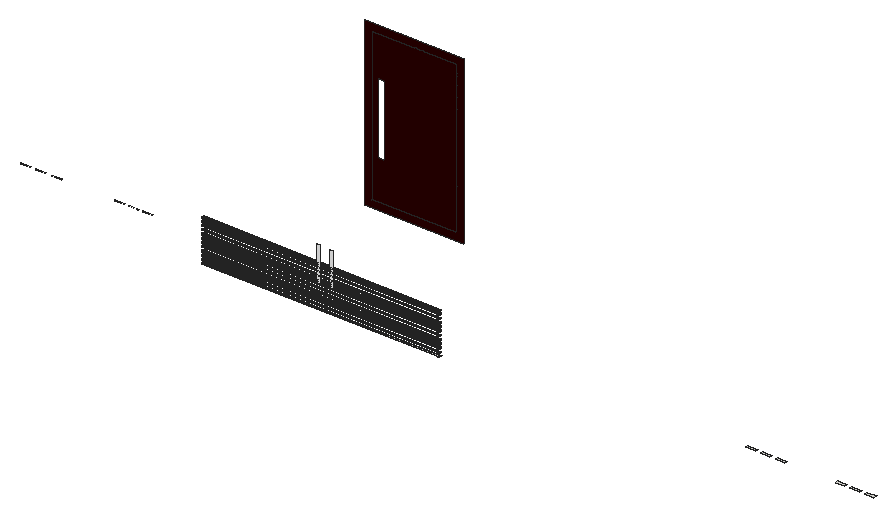
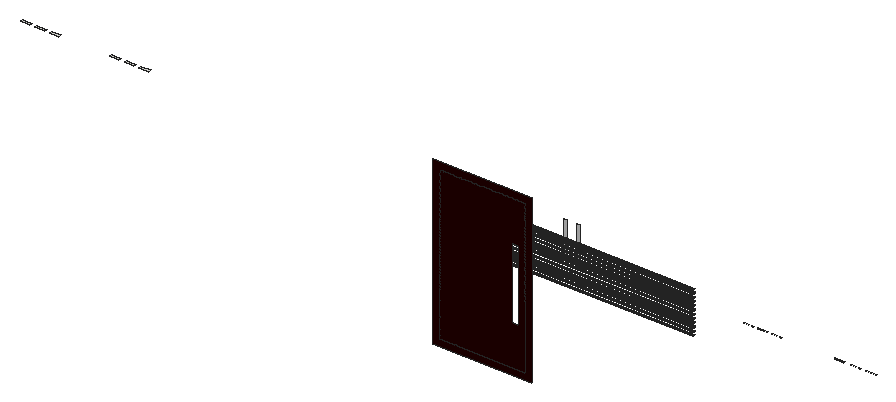
# SketchUp Ruby script. Lengths in inches.
U = 1.inch
M = Sketchup.active_model
def pt(a) = Geom::Point3d.new(a.map { |v| v * U })
def face(e, loops, mat)
  f = e.add_face(loops[0].map { |a| pt(a) })
  loops[1..].each { |l| e.add_face(l.map { |a| pt(a) }).erase! }
  f.material = f.back_material = mat if mat
  f
end
# faces: each face lists its corners as indices into pts; further lists are holes
def faces(e, pts, list, mat = nil) = list.each { |f| face(e, (f[0].is_a?(Array) ? f : [f]).map { |l| l.map { |i| pts[i] } }, mat) }
# xy, xz, yz: faces in a plane at the given z, y or x. An outline is a flat list of corners, or four numbers for a rectangle; further outlines are holes
def ring(l) = l.size == 4 ? [[l[0], l[1]], [l[2], l[1]], [l[2], l[3]], [l[0], l[3]]] : l.each_slice(2).to_a
def flat(e, list, mat, &to3) = list.each { |f| face(e, (f[0].is_a?(Array) ? f : [f]).map { |l| ring(l).map { |u, v| to3.(u, v) } }, mat) }
def xy(e, z, list, mat = nil) = flat(e, list, mat) { |x, y| [x, y, z] }
def xz(e, y, list, mat = nil) = flat(e, list, mat) { |x, z| [x, y, z] }
def yz(e, x, list, mat = nil) = flat(e, list, mat) { |y, z| [x, y, z] }
def lines(e, pts, list) = list.each { |a, b| e.add_line(pt(pts[a]), pt(pts[b])) }
# prism: a flat outline (further loops are holes) pulled along v
def prism(e, loops, v, mat = nil)
  f = face(e, loops, mat); d = Geom::Vector3d.new(v.map { |x| x * U })
  f.pushpull(f.normal.samedirection?(d) ? d.length : -d.length)
end
def box(e, o, s, mat = nil) = prism(e, [[o, [o[0] + s[0], o[1], o[2]], [o[0] + s[0], o[1] + s[1], o[2]], [o[0], o[1] + s[1], o[2]]]], [0, 0, s[2]], mat)
def at(x, y, z, deg = 0) = Geom::Transformation.translation(pt([x, y, z])) * Geom::Transformation.rotation(ORIGIN, Z_AXIS, deg.degrees)
def axes(o, x, y, z) = Geom::Transformation.new([*x, 0, *y, 0, *z, 0, *pt(o).to_a, 1])
def part(name) = M.definitions.add(name)
# library, detail: a bought-in or finely detailed component or shape, given as its bounding box
def library(name, o, s) = part(name).tap { |d| box(d.entities, o, s) }
def detail(e, o, s) = box(e.add_group.entities, o, s)
def put(e, d, t, mat = nil) = e.add_instance(d, t).tap { |i| i.material = mat if mat }
def group(e, t, mat = nil) = e.add_group.tap { |g| g.transformation = t; g.material = mat if mat }.entities
root = M.entities
M.materials.add("[0022_Maroon]").color = [43, 0, 0]
M.materials.add("[0128_White]").color = [255, 255, 255]
xy(root,190.5,[[15.39,67,40.95,69],[55.2,67,80.76,69],[98.33,67,123.89,69],[262.89,67,288.45,69],[300.83,67,326.39,69],
  [336.83,67,362.39,69]])
xy(root,214.5,[[1949.82,36,1975.38,43],[1988.38,36,2013.94,43],[2028.13,36,2053.69,43],[2185.76,36,2211.32,43],[2224.38,36,2249.94,43],
  [2262.44,36,2288.01,43]])
xz(root,71.03,[[791.39,180.6,799.64,271.47],[827.39,180.6,835.64,271.47]],"[0128_White]")
xz(root,455.71,[[[611.72,132,872.28,567.56],[629.72,150,854.28,549.56]],[[629.72,150,854.28,549.56],[645.54,254.24,665.16,443.24]]],"[0022_Maroon]")
p = [[489.6,72.78,119.6875],[489.6,72.58,119.2],[1116.35,72.58,119.2],[1116.35,72.78,119.6875],[489.6,76.45,119.2],[489.6,76.25,119.6875],
  [1116.35,76.25,119.6875],[1116.35,76.45,119.2],[489.6,73.1,120.1],[1116.35,73.1,120.1],[489.6,75.93,120.1],[1116.35,75.93,120.1],
  [489.6,73.52,120.42],[1116.35,73.52,120.42],[489.6,75.52,120.42],[1116.35,75.52,120.42],[489.6,74,120.62],[1116.35,74,120.62],
  [489.6,75.03,120.62],[1116.35,75.03,120.62],[489.6,74.52,120.6875],[1116.35,74.52,120.6875],[489.6,74,126.75],[489.6,74.52,126.6875],
  [1116.05,74.52,126.6875],[1116.05,74,126.75],[489.6,75.03,126.75],[1116.05,75.03,126.75],[489.6,73.52,126.95],[1116.05,73.52,126.95],
  [489.6,75.52,126.95],[1116.05,75.52,126.95],[489.6,73.1,127.27],[1116.05,73.1,127.27],[489.6,75.93,127.27],[1116.05,75.93,127.27],
  [489.6,72.78,127.6875],[1116.05,72.78,127.6875],[489.6,76.25,127.6875],[1116.05,76.25,127.6875],[489.6,72.58,128.17],[1116.05,72.58,128.17],
  [489.6,76.45,128.17],[1116.05,76.45,128.17],[489.6,72.52,128.6875],[1116.05,72.52,128.6875],[489.6,76.52,128.6875],[1116.05,76.52,128.6875],
  [489.6,72.58,129.2],[1116.05,72.58,129.2],[489.6,76.45,129.2],[1116.05,76.45,129.2],[489.6,72.78,129.6875],[1116.05,72.78,129.6875],
  [489.6,76.25,129.6875],[1116.05,76.25,129.6875],[489.6,73.1,130.1],[1116.05,73.1,130.1],[489.6,75.93,130.1],[1116.05,75.93,130.1],
  [489.6,73.52,130.42],[1116.05,73.52,130.42],[489.6,75.52,130.42],[1116.05,75.52,130.42],[489.6,74,130.62],[1116.05,74,130.62],
  [489.6,75.03,130.62],[1116.05,75.03,130.62],[489.6,74.52,130.6875],[1116.05,74.52,130.6875],[489.6,74,136.75],[489.6,74.52,136.6875],
  [1116.05,74.52,136.6875],[1116.05,74,136.75],[489.6,75.03,136.75],[1116.05,75.03,136.75],[489.6,73.52,136.95],[1116.05,73.52,136.95],
  [489.6,75.52,136.95],[1116.05,75.52,136.95],[489.6,73.1,137.27],[1116.05,73.1,137.27],[489.6,75.93,137.27],[1116.05,75.93,137.27],
  [489.6,72.78,137.6875],[1116.05,72.78,137.6875],[489.6,76.25,137.6875],[1116.05,76.25,137.6875],[489.6,72.58,138.17],[1116.05,72.58,138.17],
  [489.6,76.45,138.17],[1116.05,76.45,138.17],[489.6,72.52,138.6875],[1116.05,72.52,138.6875],[489.6,76.52,138.6875],[1116.05,76.52,138.6875],
  [489.6,72.58,139.2],[1116.05,72.58,139.2],[489.6,76.45,139.2],[1116.05,76.45,139.2],[489.6,72.78,139.6875],[1116.05,72.78,139.6875],
  [489.6,76.25,139.6875],[1116.05,76.25,139.6875],[489.6,73.1,140.1],[1116.05,73.1,140.1],[489.6,75.93,140.1],[1116.05,75.93,140.1],
  [489.6,73.52,140.42],[1116.05,73.52,140.42],[489.6,75.52,140.42],[1116.05,75.52,140.42],[489.6,74,140.62],[1116.05,74,140.62],
  [489.6,75.03,140.62],[1116.05,75.03,140.62],[489.6,74.52,140.6875],[1116.05,74.52,140.6875],[489.6,74,146.75],[489.6,74.52,146.6875],
  [1116.05,74.52,146.6875],[1116.05,74,146.75],[489.6,75.03,146.75],[1116.05,75.03,146.75],[489.6,73.52,146.95],[1116.05,73.52,146.95],
  [489.6,75.52,146.95],[1116.05,75.52,146.95],[489.6,73.1,147.27],[1116.05,73.1,147.27],[489.6,75.93,147.27],[1116.05,75.93,147.27],
  [489.6,72.78,147.6875],[1116.05,72.78,147.6875],[489.6,76.25,147.6875],[1116.05,76.25,147.6875],[489.6,72.58,148.17],[1116.05,72.58,148.17],
  [489.6,76.45,148.17],[1116.05,76.45,148.17],[489.6,72.52,148.6875],[1116.05,72.52,148.6875],[489.6,76.52,148.6875],[1116.05,76.52,148.6875],
  [489.6,72.58,149.2],[1116.05,72.58,149.2],[489.6,76.45,149.2],[1116.05,76.45,149.2],[489.6,72.78,149.6875],[1116.05,72.78,149.6875],
  [489.6,76.25,149.6875],[1116.05,76.25,149.6875],[489.6,73.1,150.1],[1116.05,73.1,150.1],[489.6,75.93,150.1],[1116.05,75.93,150.1],
  [489.6,73.52,150.42],[1116.05,73.52,150.42],[489.6,75.52,150.42],[1116.05,75.52,150.42],[489.6,74,150.62],[1116.05,74,150.62],
  [489.6,75.03,150.62],[1116.05,75.03,150.62],[489.6,74.52,150.6875],[1116.05,74.52,150.6875],[489.6,74,156.75],[489.6,74.52,156.6875],
  [1116.05,74.52,156.6875],[1116.05,74,156.75],[489.6,75.03,156.75],[1116.05,75.03,156.75],[489.6,73.52,156.95],[1116.05,73.52,156.95],
  [489.6,75.52,156.95],[1116.05,75.52,156.95],[489.6,73.1,157.27],[1116.05,73.1,157.27],[489.6,75.93,157.27],[1116.05,75.93,157.27],
  [489.6,72.78,157.6875],[1116.05,72.78,157.6875],[489.6,76.25,157.6875],[1116.05,76.25,157.6875],[489.6,72.58,158.17],[1116.05,72.58,158.17],
  [489.6,76.45,158.17],[1116.05,76.45,158.17],[489.6,72.52,158.6875],[1116.05,72.52,158.6875],[489.6,76.52,158.6875],[1116.05,76.52,158.6875],
  [489.6,72.58,159.2],[1116.05,72.58,159.2],[489.6,76.45,159.2],[1116.05,76.45,159.2],[489.6,72.78,159.6875],[1116.05,72.78,159.6875],
  [489.6,76.25,159.6875],[1116.05,76.25,159.6875],[489.6,73.1,160.1],[1116.05,73.1,160.1],[489.6,75.93,160.1],[1116.05,75.93,160.1],
  [489.6,73.52,160.42],[1116.05,73.52,160.42],[489.6,75.52,160.42],[1116.05,75.52,160.42],[489.6,74,160.62],[1116.05,74,160.62],
  [489.6,75.03,160.62],[1116.05,75.03,160.62],[489.6,74.52,160.6875],[1116.05,74.52,160.6875],[489.6,74,166.75],[489.6,74.52,166.6875],
  [1116.05,74.52,166.6875],[1116.05,74,166.75],[489.6,75.03,166.75],[1116.05,75.03,166.75],[489.6,73.52,166.95],[1116.05,73.52,166.95],
  [489.6,75.52,166.95],[1116.05,75.52,166.95],[489.6,73.1,167.27],[1116.05,73.1,167.27],[489.6,75.93,167.27],[1116.05,75.93,167.27],
  [489.6,72.78,167.6875],[1116.05,72.78,167.6875],[489.6,76.25,167.6875],[1116.05,76.25,167.6875],[489.6,72.58,168.17],[1116.05,72.58,168.17],
  [489.6,76.45,168.17],[1116.05,76.45,168.17],[489.6,72.52,168.6875],[1116.05,72.52,168.6875],[489.6,76.52,168.6875],[1116.05,76.52,168.6875],
  [489.6,72.58,169.2],[1116.05,72.58,169.2],[489.6,76.45,169.2],[1116.05,76.45,169.2],[489.6,72.78,169.6875],[1116.05,72.78,169.6875],
  [489.6,76.25,169.6875],[1116.05,76.25,169.6875],[489.6,73.1,170.1],[1116.05,73.1,170.1],[489.6,75.93,170.1],[1116.05,75.93,170.1],
  [489.6,73.52,170.42],[1116.05,73.52,170.42],[489.6,75.52,170.42],[1116.05,75.52,170.42],[489.6,74,170.62],[1116.05,74,170.62],
  [489.6,75.03,170.62],[1116.05,75.03,170.62],[489.6,74.52,170.6875],[1116.05,74.52,170.6875],[489.6,74,176.75],[489.6,74.52,176.6875],
  [1116.05,74.52,176.6875],[1116.05,74,176.75],[489.6,75.03,176.75],[1116.05,75.03,176.75],[489.6,73.52,176.95],[1116.05,73.52,176.95],
  [489.6,75.52,176.95],[1116.05,75.52,176.95],[489.6,73.1,177.27],[1116.05,73.1,177.27],[489.6,75.93,177.27],[1116.05,75.93,177.27],
  [489.6,72.78,177.6875],[1116.05,72.78,177.6875],[489.6,76.25,177.6875],[1116.05,76.25,177.6875],[489.6,72.58,178.17],[1116.05,72.58,178.17],
  [489.6,76.45,178.17],[1116.05,76.45,178.17],[489.6,72.52,178.6875],[1116.05,72.52,178.6875],[489.6,76.52,178.6875],[1116.05,76.52,178.6875],
  [489.6,72.58,179.2],[1116.05,72.58,179.2],[489.6,76.45,179.2],[1116.05,76.45,179.2],[489.6,72.78,179.6875],[1116.05,72.78,179.6875],
  [489.6,76.25,179.6875],[1116.05,76.25,179.6875],[489.6,73.1,180.1],[1116.05,73.1,180.1],[489.6,75.93,180.1],[1116.05,75.93,180.1],
  [489.6,73.52,180.42],[1116.05,73.52,180.42],[489.6,75.52,180.42],[1116.05,75.52,180.42],[489.6,74,180.62],[1116.05,74,180.62],
  [489.6,75.03,180.62],[1116.05,75.03,180.62],[489.6,74.52,180.6875],[1116.05,74.52,180.6875],[489.6,74,186.75],[489.6,74.52,186.6875],
  [1116.05,74.52,186.6875],[1116.05,74,186.75],[489.6,75.03,186.75],[1116.05,75.03,186.75],[489.6,73.52,186.95],[1116.05,73.52,186.95],
  [489.6,75.52,186.95],[1116.05,75.52,186.95],[489.6,73.1,187.27],[1116.05,73.1,187.27],[489.6,75.93,187.27],[1116.05,75.93,187.27],
  [489.6,72.78,187.6875],[1116.05,72.78,187.6875],[489.6,76.25,187.6875],[1116.05,76.25,187.6875],[489.6,72.58,188.17],[1116.05,72.58,188.17],
  [489.6,76.45,188.17],[1116.05,76.45,188.17],[489.6,72.52,188.6875],[1116.05,72.52,188.6875],[489.6,76.52,188.6875],[1116.05,76.52,188.6875],
  [489.6,72.58,189.2],[1116.05,72.58,189.2],[489.6,76.45,189.2],[1116.05,76.45,189.2],[489.6,72.78,189.6875],[1116.05,72.78,189.6875],
  [489.6,76.25,189.6875],[1116.05,76.25,189.6875],[489.6,73.1,190.1],[1116.05,73.1,190.1],[489.6,75.93,190.1],[1116.05,75.93,190.1],
  [489.6,73.52,190.42],[1116.05,73.52,190.42],[489.6,75.52,190.42],[1116.05,75.52,190.42],[489.6,74,190.62],[1116.05,74,190.62],
  [489.6,75.03,190.62],[1116.05,75.03,190.62],[489.6,74.52,190.6875],[1116.05,74.52,190.6875],[489.6,74,196.75],[489.6,74.52,196.6875],
  [1116.05,74.52,196.6875],[1116.05,74,196.75],[489.6,75.03,196.75],[1116.05,75.03,196.75],[489.6,73.52,196.95],[1116.05,73.52,196.95],
  [489.6,75.52,196.95],[1116.05,75.52,196.95],[489.6,73.1,197.27],[1116.05,73.1,197.27],[489.6,75.93,197.27],[1116.05,75.93,197.27],
  [489.6,72.78,197.6875],[1116.05,72.78,197.6875],[489.6,76.25,197.6875],[1116.05,76.25,197.6875],[489.6,72.58,198.17],[1116.05,72.58,198.17],
  [489.6,76.45,198.17],[1116.05,76.45,198.17],[489.6,72.52,198.6875],[1116.05,72.52,198.6875],[489.6,76.52,198.6875],[1116.05,76.52,198.6875],
  [489.6,72.58,199.2],[1116.05,72.58,199.2],[489.6,76.45,199.2],[1116.05,76.45,199.2],[489.6,72.78,199.6875],[1116.05,72.78,199.6875],
  [489.6,76.25,199.6875],[1116.05,76.25,199.6875],[489.6,73.1,200.1],[1116.05,73.1,200.1],[489.6,75.93,200.1],[1116.05,75.93,200.1],
  [489.6,73.52,200.42],[1116.05,73.52,200.42],[489.6,75.52,200.42],[1116.05,75.52,200.42],[489.6,74,200.62],[1116.05,74,200.62],
  [489.6,75.03,200.62],[1116.05,75.03,200.62],[489.6,74.52,200.6875],[1116.05,74.52,200.6875],[489.6,74,206.75],[489.6,74.52,206.6875],
  [1116.05,74.52,206.6875],[1116.05,74,206.75],[489.6,75.03,206.75],[1116.05,75.03,206.75],[489.6,73.52,206.95],[1116.05,73.52,206.95],
  [489.6,75.52,206.95],[1116.05,75.52,206.95],[489.6,73.1,207.27],[1116.05,73.1,207.27],[489.6,75.93,207.27],[1116.05,75.93,207.27],
  [489.6,72.78,207.6875],[1116.05,72.78,207.6875],[489.6,76.25,207.6875],[1116.05,76.25,207.6875],[489.6,72.58,208.17],[1116.05,72.58,208.17],
  [489.6,76.45,208.17],[1116.05,76.45,208.17],[489.6,72.52,208.6875],[1116.05,72.52,208.6875],[489.6,76.52,208.6875],[1116.05,76.52,208.6875],
  [489.6,72.58,209.2],[1116.05,72.58,209.2],[489.6,76.45,209.2],[1116.05,76.45,209.2],[489.6,72.78,209.6875],[1116.05,72.78,209.6875],
  [489.6,76.25,209.6875],[1116.05,76.25,209.6875],[489.6,73.1,210.1],[1116.05,73.1,210.1],[489.6,75.93,210.1],[1116.05,75.93,210.1],
  [489.6,73.52,210.42],[1116.05,73.52,210.42],[489.6,75.52,210.42],[1116.05,75.52,210.42],[489.6,74,210.62],[1116.05,74,210.62],
  [489.6,75.03,210.62],[1116.05,75.03,210.62],[489.6,74.52,210.6875],[1116.05,74.52,210.6875],[489.6,74,216.75],[489.6,74.52,216.6875],
  [1116.05,74.52,216.6875],[1116.05,74,216.75],[489.6,75.03,216.75],[1116.05,75.03,216.75],[489.6,73.52,216.95],[1116.05,73.52,216.95],
  [489.6,75.52,216.95],[1116.05,75.52,216.95],[489.6,73.1,217.27],[1116.05,73.1,217.27],[489.6,75.93,217.27],[1116.05,75.93,217.27],
  [489.6,72.78,217.6875],[1116.05,72.78,217.6875],[489.6,76.25,217.6875],[1116.05,76.25,217.6875],[489.6,72.58,218.17],[1116.05,72.58,218.17],
  [489.6,76.45,218.17],[1116.05,76.45,218.17],[489.6,72.52,218.6875],[1116.05,72.52,218.6875],[489.6,76.52,218.6875],[1116.05,76.52,218.6875],
  [489.6,72.58,219.2],[1116.05,72.58,219.2],[489.6,76.45,219.2],[1116.05,76.45,219.2],[489.6,72.78,219.6875],[1116.05,72.78,219.6875],
  [489.6,76.25,219.6875],[1116.05,76.25,219.6875],[489.6,73.1,220.1],[1116.05,73.1,220.1],[489.6,75.93,220.1],[1116.05,75.93,220.1],
  [489.6,73.52,220.42],[1116.05,73.52,220.42],[489.6,75.52,220.42],[1116.05,75.52,220.42],[489.6,74,220.62],[1116.05,74,220.62],
  [489.6,75.03,220.62],[1116.05,75.03,220.62],[489.6,74.52,220.6875],[1116.05,74.52,220.6875],[489.6,74,226.75],[489.6,74.52,226.6875],
  [1116.05,74.52,226.6875],[1116.05,74,226.75],[489.6,75.03,226.75],[1116.05,75.03,226.75],[489.6,73.52,226.95],[1116.05,73.52,226.95],
  [489.6,75.52,226.95],[1116.05,75.52,226.95],[489.6,73.1,227.27],[1116.05,73.1,227.27],[489.6,75.93,227.27],[1116.05,75.93,227.27],
  [489.6,72.78,227.6875],[1116.05,72.78,227.6875],[489.6,76.25,227.6875],[1116.05,76.25,227.6875],[489.6,72.58,228.17],[1116.05,72.58,228.17],
  [489.6,76.45,228.17],[1116.05,76.45,228.17],[489.6,72.52,228.6875],[1116.05,72.52,228.6875],[489.6,76.52,228.6875],[1116.05,76.52,228.6875]]
faces(root,p,[[0,1,2,3],[4,5,6,7],[8,0,3,9],[5,10,11,6],[12,8,9,13],[10,14,15,11],[16,12,13,17],[14,18,19,15],
  [20,16,17,21],[18,20,21,19],[22,23,24,25],[23,26,27,24],[28,22,25,29],[26,30,31,27],[32,28,29,33],[30,34,35,31],
  [36,32,33,37],[34,38,39,35],[40,36,37,41],[38,42,43,39],[44,40,41,45],[42,46,47,43],[48,44,45,49],[46,50,51,47],
  [52,48,49,53],[50,54,55,51],[56,52,53,57],[54,58,59,55],[60,56,57,61],[58,62,63,59],[64,60,61,65],[62,66,67,63],
  [68,64,65,69],[66,68,69,67],[70,71,72,73],[71,74,75,72],[76,70,73,77],[74,78,79,75],[80,76,77,81],[78,82,83,79],
  [84,80,81,85],[82,86,87,83],[88,84,85,89],[86,90,91,87],[92,88,89,93],[90,94,95,91],[96,92,93,97],[94,98,99,95],
  [100,96,97,101],[98,102,103,99],[104,100,101,105],[102,106,107,103],[108,104,105,109],[106,110,111,107],[112,108,109,113],[110,114,115,111],
  [116,112,113,117],[114,116,117,115],[118,119,120,121],[119,122,123,120],[124,118,121,125],[122,126,127,123],[128,124,125,129],[126,130,131,127],
  [132,128,129,133],[130,134,135,131],[136,132,133,137],[134,138,139,135],[140,136,137,141],[138,142,143,139],[144,140,141,145],[142,146,147,143],
  [148,144,145,149],[146,150,151,147],[152,148,149,153],[150,154,155,151],[156,152,153,157],[154,158,159,155],[160,156,157,161],[158,162,163,159],
  [164,160,161,165],[162,164,165,163],[166,167,168,169],[167,170,171,168],[172,166,169,173],[170,174,175,171],[176,172,173,177],[174,178,179,175],
  [180,176,177,181],[178,182,183,179],[184,180,181,185],[182,186,187,183],[188,184,185,189],[186,190,191,187],[192,188,189,193],[190,194,195,191],
  [196,192,193,197],[194,198,199,195],[200,196,197,201],[198,202,203,199],[204,200,201,205],[202,206,207,203],[208,204,205,209],[206,210,211,207],
  [212,208,209,213],[210,212,213,211],[214,215,216,217],[215,218,219,216],[220,214,217,221],[218,222,223,219],[224,220,221,225],[222,226,227,223],
  [228,224,225,229],[226,230,231,227],[232,228,229,233],[230,234,235,231],[236,232,233,237],[234,238,239,235],[240,236,237,241],[238,242,243,239],
  [244,240,241,245],[242,246,247,243],[248,244,245,249],[246,250,251,247],[252,248,249,253],[250,254,255,251],[256,252,253,257],[254,258,259,255],
  [260,256,257,261],[258,260,261,259],[262,263,264,265],[263,266,267,264],[268,262,265,269],[266,270,271,267],[272,268,269,273],[270,274,275,271],
  [276,272,273,277],[274,278,279,275],[280,276,277,281],[278,282,283,279],[284,280,281,285],[282,286,287,283],[288,284,285,289],[286,290,291,287],
  [292,288,289,293],[290,294,295,291],[296,292,293,297],[294,298,299,295],[300,296,297,301],[298,302,303,299],[304,300,301,305],[302,306,307,303],
  [308,304,305,309],[306,308,309,307],[310,311,312,313],[311,314,315,312],[316,310,313,317],[314,318,319,315],[320,316,317,321],[318,322,323,319],
  [324,320,321,325],[322,326,327,323],[328,324,325,329],[326,330,331,327],[332,328,329,333],[330,334,335,331],[336,332,333,337],[334,338,339,335],
  [340,336,337,341],[338,342,343,339],[344,340,341,345],[342,346,347,343],[348,344,345,349],[346,350,351,347],[352,348,349,353],[350,354,355,351],
  [356,352,353,357],[354,356,357,355],[358,359,360,361],[359,362,363,360],[364,358,361,365],[362,366,367,363],[368,364,365,369],[366,370,371,367],
  [372,368,369,373],[370,374,375,371],[376,372,373,377],[374,378,379,375],[380,376,377,381],[378,382,383,379],[384,380,381,385],[382,386,387,383],
  [388,384,385,389],[386,390,391,387],[392,388,389,393],[390,394,395,391],[396,392,393,397],[394,398,399,395],[400,396,397,401],[398,402,403,399],
  [404,400,401,405],[402,404,405,403],[406,407,408,409],[407,410,411,408],[412,406,409,413],[410,414,415,411],[416,412,413,417],[414,418,419,415],
  [420,416,417,421],[418,422,423,419],[424,420,421,425],[422,426,427,423],[428,424,425,429],[426,430,431,427],[432,428,429,433],[430,434,435,431],
  [436,432,433,437],[434,438,439,435],[440,436,437,441],[438,442,443,439],[444,440,441,445],[442,446,447,443],[448,444,445,449],[446,450,451,447],
  [452,448,449,453],[450,452,453,451],[454,455,456,457],[455,458,459,456],[460,454,457,461],[458,462,463,459],[464,460,461,465],[462,466,467,463],
  [468,464,465,469],[466,470,471,467],[472,468,469,473],[470,474,475,471],[476,472,473,477],[474,478,479,475],[480,476,477,481],[478,482,483,479],
  [484,480,481,485],[482,486,487,483],[488,484,485,489],[486,490,491,487],[492,488,489,493],[490,494,495,491],[496,492,493,497],[494,498,499,495],
  [500,496,497,501],[498,500,501,499],[502,503,504,505],[503,506,507,504],[508,502,505,509],[506,510,511,507],[512,508,509,513],[510,514,515,511],
  [516,512,513,517],[514,518,519,515],[520,516,517,521],[518,522,523,519],[524,520,521,525],[522,526,527,523]])
